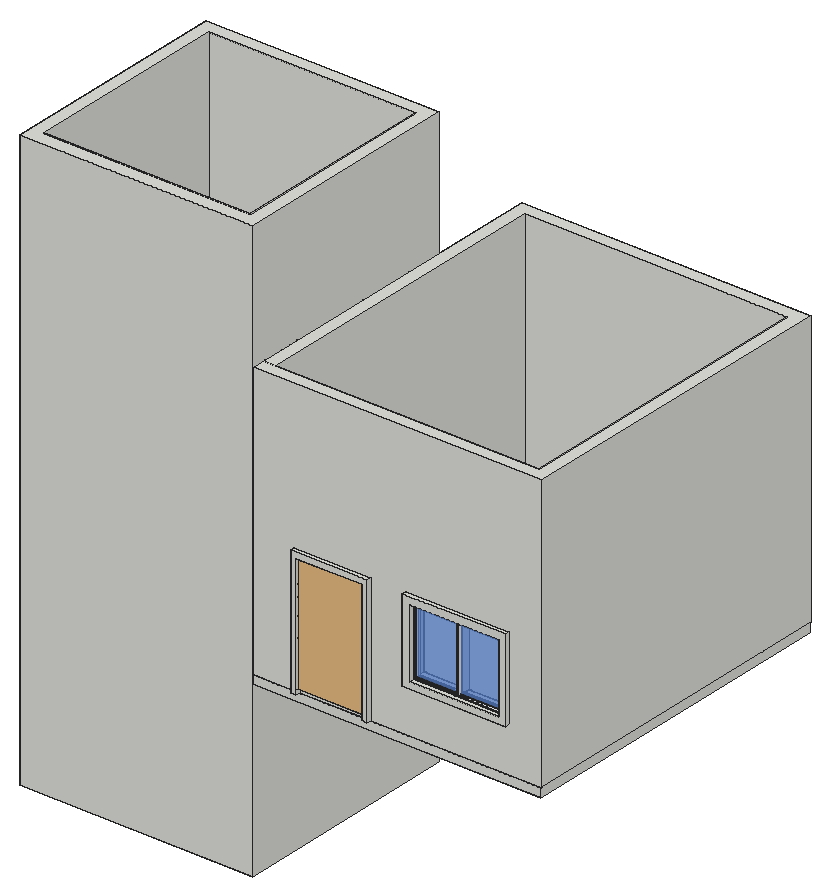
# SketchUp Ruby script. Lengths in inches.
U = 1.inch
M = Sketchup.active_model
def pt(a) = Geom::Point3d.new(a.map { |v| v * U })
def face(e, loops, mat)
  f = e.add_face(loops[0].map { |a| pt(a) })
  loops[1..].each { |l| e.add_face(l.map { |a| pt(a) }).erase! }
  f.material = f.back_material = mat if mat
  f
end
# faces: each face lists its corners as indices into pts; further lists are holes
def faces(e, pts, list, mat = nil) = list.each { |f| face(e, (f[0].is_a?(Array) ? f : [f]).map { |l| l.map { |i| pts[i] } }, mat) }
# xy, xz, yz: faces in a plane at the given z, y or x. An outline is a flat list of corners, or four numbers for a rectangle; further outlines are holes
def ring(l) = l.size == 4 ? [[l[0], l[1]], [l[2], l[1]], [l[2], l[3]], [l[0], l[3]]] : l.each_slice(2).to_a
def flat(e, list, mat, &to3) = list.each { |f| face(e, (f[0].is_a?(Array) ? f : [f]).map { |l| ring(l).map { |u, v| to3.(u, v) } }, mat) }
def xy(e, z, list, mat = nil) = flat(e, list, mat) { |x, y| [x, y, z] }
def xz(e, y, list, mat = nil) = flat(e, list, mat) { |x, z| [x, y, z] }
def yz(e, x, list, mat = nil) = flat(e, list, mat) { |y, z| [x, y, z] }
def lines(e, pts, list) = list.each { |a, b| e.add_line(pt(pts[a]), pt(pts[b])) }
# prism: a flat outline (further loops are holes) pulled along v
def prism(e, loops, v, mat = nil)
  f = face(e, loops, mat); d = Geom::Vector3d.new(v.map { |x| x * U })
  f.pushpull(f.normal.samedirection?(d) ? d.length : -d.length)
end
def box(e, o, s, mat = nil) = prism(e, [[o, [o[0] + s[0], o[1], o[2]], [o[0] + s[0], o[1] + s[1], o[2]], [o[0], o[1] + s[1], o[2]]]], [0, 0, s[2]], mat)
def at(x, y, z, deg = 0) = Geom::Transformation.translation(pt([x, y, z])) * Geom::Transformation.rotation(ORIGIN, Z_AXIS, deg.degrees)
def axes(o, x, y, z) = Geom::Transformation.new([*x, 0, *y, 0, *z, 0, *pt(o).to_a, 1])
def part(name) = M.definitions.add(name)
# library, detail: a bought-in or finely detailed component or shape, given as its bounding box
def library(name, o, s) = part(name).tap { |d| box(d.entities, o, s) }
def detail(e, o, s) = box(e.add_group.entities, o, s)
def put(e, d, t, mat = nil) = e.add_instance(d, t).tap { |i| i.material = mat if mat }
def group(e, t, mat = nil) = e.add_group.tap { |g| g.transformation = t; g.material = mat if mat }.entities
root = M.entities
M.materials.add("[Metal Silver]").color = [234, 233, 238]
M.materials.add("[Translucent Glass Blue]").color = [100, 149, 237]
M.materials["[Translucent Glass Blue]"].alpha = 0.5
c1 = part("Group1\#1")
prism(c1.entities,[[[84,247.9375,0],[246,247.9375,0],[246,85.9375,0],[84,85.9375,0]],[[237,94.9375,0],[237,238.9375,0],[93,238.9375,0],[93,94.9375,0]]],[0,0,405.6875])
c2 = library("Group\#5",[0,0,0],[45.42,10.47,82])
c3 = part("Group12\#1")
xy(c3.entities,126,[[274.58,235.9375,274.58,238.9375,246,238.9375,246,247.9375,438,247.9375,438,463.9375,255,463.9375,255,247.9375,246,247.9375,246,472.9375,447,472.9375,447,238.9375,328,238.9375,328,235.9375,324,235.9375,324,238.9375,278.58,238.9375,278.58,235.9375]])
xy(c3.entities,129,[[278.58,238.9375,324,247.9375]])
xy(c3.entities,157.39,[[352.34,235.9375,424.28,238.9375]])
xy(c3.entities,162,[[357.34,235.9375,419.67,247.9375]])
xy(c3.entities,210,[[357.34,235.9375,419.67,247.9375]])
xy(c3.entities,211,[[278.58,235.9375,324,247.9375]])
xy(c3.entities,215,[[274.58,235.9375,328,238.9375],[352.34,235.9375,424.28,238.9375]])
xy(c3.entities,317.5,[[246,238.9375,447,238.9375,447,472.9375,246,472.9375,246,247.9375,255,247.9375,255,463.9375,438,463.9375,438,247.9375,246,247.9375]])
xz(c3.entities,235.9375,[[274.58,126,278.58,126,278.58,211,324,211,324,126,328,126,328,215,274.58,215],[[352.34,157.39,424.28,215],[357.34,162,419.67,210]]])
xz(c3.entities,238.9375,[[[246,126,274.58,126,274.58,215,328,215,328,126,447,126,447,317.5,246,317.5],[352.34,157.39,424.28,215]],[278.58,126,324,129]])
xz(c3.entities,247.9375,[[246,126,255,246],[[255,126,438,317.5],[278.58,129,324,211],[357.34,162,419.67,210]],[246,246,255,317.5]])
xz(c3.entities,463.9375,[[255,126,438,317.5]])
xz(c3.entities,472.9375,[[246,126,447,317.5]])
yz(c3.entities,246,[[238.9375,126,247.9375,317.5],[247.9375,126,472.9375,317.5]])
yz(c3.entities,255,[[247.9375,126,463.9375,317.5]])
yz(c3.entities,274.58,[[235.9375,126,238.9375,215]])
yz(c3.entities,278.58,[[235.9375,126,238.9375,129],[235.9375,129,247.9375,211]])
yz(c3.entities,324,[[235.9375,126,238.9375,129],[235.9375,129,247.9375,211]])
yz(c3.entities,328,[[235.9375,126,238.9375,215]])
yz(c3.entities,352.34,[[235.9375,157.39,238.9375,215]])
yz(c3.entities,357.34,[[235.9375,162,247.9375,210]])
yz(c3.entities,419.67,[[235.9375,162,247.9375,210]])
yz(c3.entities,424.28,[[235.9375,157.39,238.9375,215]])
yz(c3.entities,438,[[247.9375,126,463.9375,317.5]])
yz(c3.entities,447,[[238.9375,126,472.9375,317.5]])
put(c3.entities,c2,at(278.58,237.47,129))
c4 = part("Group19\#2")
box(c4.entities,[1.02,-2.16,1.02],[60.29,0.63,45.96])
put(root,c1,at(-84,-82.9375,0))
g1 = group(root,at(162,2.625,120))
box(g1,[0,0,0],[201,234,6])
put(root,c3,at(-84,-235.9375,0))
g2 = group(root,at(273.34,3,162))
put(g2,c4,at(62.33,0,0,180),"[Translucent Glass Blue]")
g3 = group(g2,at(62.33,0,0,180),"[Metal Silver]")
xy(g3,0,[[0,-9,30.34,0],[30.34,-9,31.99,0],[31.99,-9,62.33,0]])
xy(g3,0.83,[[0.83,-8.93,30.34,-4.61],[31.99,-8.93,61.5,-4.61]])
xy(g3,1.02,[[1.02,-3.3125,30.34,-2.16],[30.34,-3.3125,31.99,-2.16],[31.99,-3.3125,61.31,-2.16]])
xy(g3,1.61,[[1.61,-2.16,30.34,-1.8],[31.99,-2.16,60.72,-1.8]])
xy(g3,1.65,[[1.65,-3.46,30.34,-3.3125],[31.99,-3.46,60.68,-3.3125]])
xy(g3,46.35,[[1.65,-3.46,30.34,-3.3125],[31.99,-3.46,60.68,-3.3125]])
xy(g3,46.39,[[1.61,-2.16,30.34,-1.8],[31.99,-2.16,60.72,-1.8]])
xy(g3,46.98,[[1.02,-3.3125,30.34,-2.16],[30.34,-3.3125,31.99,-2.16],[31.99,-3.3125,61.31,-2.16]])
xy(g3,47.17,[[0.83,-8.93,30.34,-4.61],[31.99,-8.93,61.5,-4.61]])
xy(g3,48,[[0,-9,30.34,0],[30.34,-9,31.99,0],[31.99,-9,62.33,0]])
xz(g3,-9.07,[[0.04,0.04,30.34,0.04,30.34,0.75,0.75,0.75,0.75,47.25,30.34,47.25,30.34,47.96,0.04,47.96],[30.34,0.04,31.99,47.96],[31.99,0.04,62.29,0.04,62.29,47.96,31.99,47.96,31.99,47.25,61.58,47.25,61.58,0.75,31.99,0.75]])
xz(g3,-4.61,[[0.83,0.83,30.34,0.83,30.34,1.5,1.5,1.5,1.5,46.5,30.34,46.5,30.34,47.17,0.83,47.17],[31.99,0.83,61.5,0.83,61.5,47.17,31.99,47.17,31.99,46.5,60.83,46.5,60.83,1.5,31.99,1.5]])
xz(g3,-3.3125,[[1.02,1.02,1.02,46.98,30.34,46.98,30.34,46.35,1.65,46.35,1.65,1.65,30.34,1.65,30.34,1.02],[30.34,1.02,31.99,46.98],[31.99,1.02,31.99,1.65,60.68,1.65,60.68,46.35,31.99,46.35,31.99,46.98,61.31,46.98,61.31,1.02]])
xz(g3,-2.16,[[1.02,1.02,30.34,1.02,30.34,1.61,1.61,1.61,1.61,46.39,30.34,46.39,30.34,46.98,1.02,46.98],[30.34,1.02,31.99,46.98],[31.99,1.02,61.31,1.02,61.31,46.98,31.99,46.98,31.99,46.39,60.72,46.39,60.72,1.61,31.99,1.61]])
xz(g3,-1.8,[[0.83,0.83,0.83,47.17,30.34,47.17,30.34,46.39,1.61,46.39,1.61,1.61,30.34,1.61,30.34,0.83],[31.99,0.83,31.99,1.61,60.72,1.61,60.72,46.39,31.99,46.39,31.99,47.17,61.5,47.17,61.5,0.83]])
xz(g3,-0.36,[[0.59,0.59,0.59,47.41,30.34,47.41,30.34,47.21,0.79,47.21,0.79,0.79,30.34,0.79,30.34,0.59],[31.99,0.59,31.99,0.79,61.54,0.79,61.54,47.21,31.99,47.21,31.99,47.41,61.74,47.41,61.74,0.59]])
xz(g3,0,[[0,0,0,48,30.34,48,30.34,47.61,0.39,47.61,0.39,0.39,30.34,0.39,30.34,0],[30.34,0,31.99,48],[31.99,0,31.99,0.39,61.9375,0.39,61.9375,47.61,31.99,47.61,31.99,48,62.33,48,62.33,0]])
yz(g3,0,[[-9,0,0,48]])
yz(g3,0.83,[[-8.93,0.83,-4.61,47.17]])
yz(g3,1.02,[[-3.3125,1.02,-2.16,46.98]])
yz(g3,1.61,[[-2.16,1.61,-1.8,46.39]])
yz(g3,1.65,[[-3.46,1.65,-3.3125,46.35]])
yz(g3,30.34,[[-9,0,0,0,0,0.39,-0.36,0.59,-0.36,0.79,-1.8,0.83,-1.8,1.61,-2.16,1.61,-2.16,1.02,-3.3125,1.02,-3.3125,1.65,-3.46,1.65,-4.61,1.5,-4.61,0.83,-8.93,0.83,-9.07,0.75,-9.07,0.04],[[-9,0,-9.07,0.04,-9.07,47.96,-9,48,0,48,0,0],[-3.3125,1.02,-2.16,46.98]],[-3.46,46.35,-3.3125,46.35,-3.3125,46.98,-2.16,46.98,-2.16,46.39,-1.8,46.39,-1.8,47.17,-0.36,47.21,-0.36,47.41,0,47.61,0,48,-9,48,-9.07,47.96,-9.07,47.25,-8.93,47.17,-4.61,47.17,-4.61,46.5]])
yz(g3,31.99,[[-9,0,-9.07,0.04,-9.07,0.75,-8.93,0.83,-4.61,0.83,-4.61,1.5,-3.46,1.65,-3.3125,1.65,-3.3125,1.02,-2.16,1.02,-2.16,1.61,-1.8,1.61,-1.8,0.83,-0.36,0.79,-0.36,0.59,0,0.39,0,0],[[-9,0,0,0,0,48,-9,48,-9.07,47.96,-9.07,0.04],[-3.3125,1.02,-2.16,46.98]],[-3.46,46.35,-4.61,46.5,-4.61,47.17,-8.93,47.17,-9.07,47.25,-9.07,47.96,-9,48,0,48,0,47.61,-0.36,47.41,-0.36,47.21,-1.8,47.17,-1.8,46.39,-2.16,46.39,-2.16,46.98,-3.3125,46.98,-3.3125,46.35]])
yz(g3,60.68,[[-3.46,1.65,-3.3125,46.35]])
yz(g3,60.72,[[-2.16,1.61,-1.8,46.39]])
yz(g3,61.31,[[-3.3125,1.02,-2.16,46.98]])
yz(g3,61.5,[[-8.93,0.83,-4.61,47.17]])
yz(g3,62.33,[[-9,0,0,48]])
p = [[30.34,-9,0],[30.34,-9.07,0.04],[0.04,-9.07,0.04],[0,-9,0],[0.04,-9.07,47.96],[0,-9,48],
  [31.99,-9,0],[31.99,-9.07,0.04],[62.33,-9,0],[62.29,-9.07,0.04],[62.33,-9,48],[62.29,-9.07,47.96],
  [30.34,-0.36,0.59],[30.34,0,0.39],[0.39,0,0.39],[0.59,-0.36,0.59],[0.39,0,47.61],[0.59,-0.36,47.41],
  [31.99,0,0.39],[31.99,-0.36,0.59],[61.74,-0.36,0.59],[61.9375,0,0.39],[61.74,-0.36,47.41],[61.9375,0,47.61],
  [30.34,-9.07,0.75],[30.34,-8.93,0.83],[0.83,-8.93,0.83],[0.75,-9.07,0.75],[0.83,-8.93,47.17],[0.75,-9.07,47.25],
  [31.99,-8.93,0.83],[31.99,-9.07,0.75],[61.58,-9.07,0.75],[61.5,-8.93,0.83],[61.58,-9.07,47.25],[61.5,-8.93,47.17],
  [30.34,-1.8,0.83],[30.34,-0.36,0.79],[0.79,-0.36,0.79],[0.83,-1.8,0.83],[0.79,-0.36,47.21],[0.83,-1.8,47.17],
  [31.99,-0.36,0.79],[31.99,-1.8,0.83],[61.5,-1.8,0.83],[61.54,-0.36,0.79],[61.5,-1.8,47.17],[61.54,-0.36,47.21],
  [30.34,-4.61,1.5],[30.34,-3.46,1.65],[1.65,-3.46,1.65],[1.5,-4.61,1.5],[1.65,-3.46,46.35],[1.5,-4.61,46.5],
  [31.99,-3.46,1.65],[31.99,-4.61,1.5],[60.83,-4.61,1.5],[60.68,-3.46,1.65],[60.83,-4.61,46.5],[60.68,-3.46,46.35],
  [30.34,-3.46,46.35],[30.34,-4.61,46.5],[31.99,-4.61,46.5],[31.99,-3.46,46.35],[30.34,-8.93,47.17],[30.34,-9.07,47.25],
  [31.99,-9.07,47.25],[31.99,-8.93,47.17],[30.34,-0.36,47.21],[30.34,-1.8,47.17],[31.99,-1.8,47.17],[31.99,-0.36,47.21],
  [30.34,0,47.61],[30.34,-0.36,47.41],[31.99,-0.36,47.41],[31.99,0,47.61],[30.34,-9.07,47.96],[30.34,-9,48],
  [31.99,-9.07,47.96],[31.99,-9,48]]
faces(g3,p,[[0,1,2,3],[3,2,4,5],[6,7,1,0],[7,6,8,9],[9,8,10,11],[12,13,14,15],[15,14,16,17],[18,19,20,21],
  [21,20,22,23],[24,25,26,27],[27,26,28,29],[30,31,32,33],[33,32,34,35],[36,37,38,39],[39,38,40,41],[42,43,44,45],
  [45,44,46,47],[48,49,50,51],[51,50,52,53],[54,55,56,57],[57,56,58,59],[53,52,60,61],[59,58,62,63],[29,28,64,65],
  [35,34,66,67],[41,40,68,69],[47,46,70,71],[17,16,72,73],[23,22,74,75],[5,4,76,77],[78,79,77,76],[11,10,79,78]])
